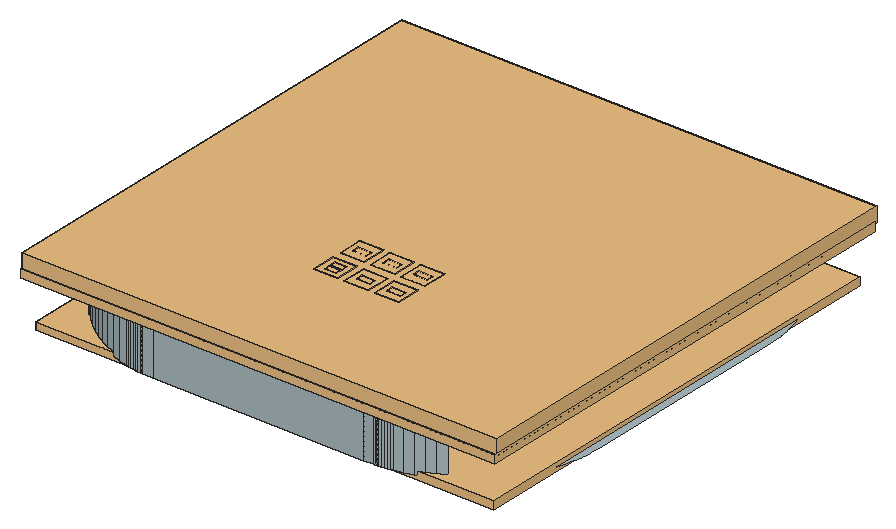
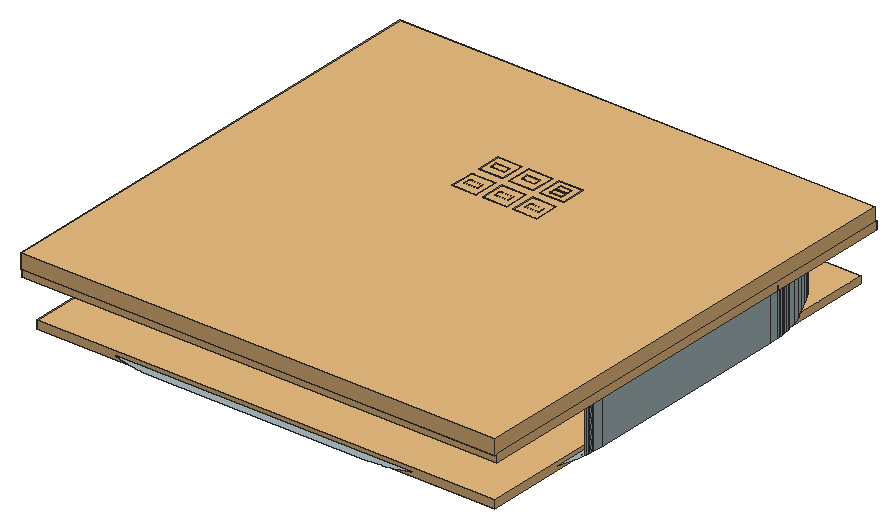
# SketchUp Ruby script. Lengths in inches.
U = 1.inch
M = Sketchup.active_model
def pt(a) = Geom::Point3d.new(a.map { |v| v * U })
def face(e, loops, mat)
  f = e.add_face(loops[0].map { |a| pt(a) })
  loops[1..].each { |l| e.add_face(l.map { |a| pt(a) }).erase! }
  f.material = f.back_material = mat if mat
  f
end
# faces: each face lists its corners as indices into pts; further lists are holes
def faces(e, pts, list, mat = nil) = list.each { |f| face(e, (f[0].is_a?(Array) ? f : [f]).map { |l| l.map { |i| pts[i] } }, mat) }
# xy, xz, yz: faces in a plane at the given z, y or x. An outline is a flat list of corners, or four numbers for a rectangle; further outlines are holes
def ring(l) = l.size == 4 ? [[l[0], l[1]], [l[2], l[1]], [l[2], l[3]], [l[0], l[3]]] : l.each_slice(2).to_a
def flat(e, list, mat, &to3) = list.each { |f| face(e, (f[0].is_a?(Array) ? f : [f]).map { |l| ring(l).map { |u, v| to3.(u, v) } }, mat) }
def xy(e, z, list, mat = nil) = flat(e, list, mat) { |x, y| [x, y, z] }
def xz(e, y, list, mat = nil) = flat(e, list, mat) { |x, z| [x, y, z] }
def yz(e, x, list, mat = nil) = flat(e, list, mat) { |y, z| [x, y, z] }
def lines(e, pts, list) = list.each { |a, b| e.add_line(pt(pts[a]), pt(pts[b])) }
# prism: a flat outline (further loops are holes) pulled along v
def prism(e, loops, v, mat = nil)
  f = face(e, loops, mat); d = Geom::Vector3d.new(v.map { |x| x * U })
  f.pushpull(f.normal.samedirection?(d) ? d.length : -d.length)
end
def box(e, o, s, mat = nil) = prism(e, [[o, [o[0] + s[0], o[1], o[2]], [o[0] + s[0], o[1] + s[1], o[2]], [o[0], o[1] + s[1], o[2]]]], [0, 0, s[2]], mat)
def at(x, y, z, deg = 0) = Geom::Transformation.translation(pt([x, y, z])) * Geom::Transformation.rotation(ORIGIN, Z_AXIS, deg.degrees)
def axes(o, x, y, z) = Geom::Transformation.new([*x, 0, *y, 0, *z, 0, *pt(o).to_a, 1])
def part(name) = M.definitions.add(name)
# library, detail: a bought-in or finely detailed component or shape, given as its bounding box
def library(name, o, s) = part(name).tap { |d| box(d.entities, o, s) }
def detail(e, o, s) = box(e.add_group.entities, o, s)
def put(e, d, t, mat = nil) = e.add_instance(d, t).tap { |i| i.material = mat if mat }
def group(e, t, mat = nil) = e.add_group.tap { |g| g.transformation = t; g.material = mat if mat }.entities
root = M.entities
M.materials.add("11").color = [255, 255, 255]
M.materials.add("26").color = [169, 186, 191]
c1 = library("Group103",[37538.96,7398.86,1636.89],[6.69,3.33,0.23])
c2 = library("Group97",[37538.89,7403.08,1636.87],[6.82,3.31,0.23])
c3 = library("Group98",[37538.36,7420.16,1636.8],[7.89,3.87,0.23])
c4 = library("om.cn_51",[-14089.91,-120000,166752.75],[16176.5,10000,4589.03])
c5 = library("om.cn_51698238",[-12277.97,-120000,175247.47],[24687.75,10000,11950.5])
c6 = library("Group104",[37556.32,7400.57,1636.88],[7.75,3.92,0.23])
c7 = library("Group99",[37556.29,7420.12,1636.8],[7.81,3.89,0.23])
c8 = library("Group113",[-159,-159,0],[318,318,8.4])
c9 = library("Group111",[-148.91,-148.91,209.88],[297.82,297.82,5])
c10 = library("Group59",[-149.91,-149.91,265.34],[299.82,299.82,4.68])
c11 = library("om.cn_51268574",[-7425.4375,-120000,166763.1875],[21515.3125,10000,4564.15])
c12 = library("Group105",[37574.14,7400.59,1636.88],[7.9,3.89,0.23])
c13 = library("Group101",[37574.11,7420.12,1636.8],[7.96,3.91,0.23])
xy(root,90.6622,[[[290.4563,4.7461,290.2394,4.7537,290.2089,4.756,290.1785,4.7586,290.148,4.7615,290.1176,4.7648,290.0873,4.7683,290.0569,4.7721,290.0266,4.7763,289.9968,4.7806,289.9669,4.7853,289.9371,4.7903,289.9074,4.7956,289.8777,4.8012,289.848,4.8071,289.8185,4.8133,289.6154,4.8641,289.418,4.9284,289.2268,5.0055,289.0422,5.095,288.8648,5.1964,288.6951,5.309,288.5336,5.4324,288.3809,5.5662,288.2374,5.7097,288.1036,5.8624,287.9802,6.0239,287.8676,6.1936,287.7662,6.371,287.6768,6.5556,287.5996,6.7468,287.5353,6.9442,287.4845,7.1473,287.4783,7.1768,287.4724,7.2065,287.4668,7.2362,287.4615,7.2659,287.4565,7.2957,287.4519,7.3255,287.4475,7.3554,287.4433,7.3857,287.4395,7.4161,287.436,7.4464,287.4327,7.4768,287.4298,7.5073,287.4272,7.5377,287.4249,7.5682,287.4173,7.7851,287.4173,12.6889,287.4249,12.9057,287.4272,12.9362,287.4298,12.9667,287.4327,12.9971,287.436,13.0275,287.4395,13.0579,287.4433,13.0882,287.4475,13.1185,287.4519,13.1484,287.4565,13.1782,287.4615,13.208,287.4668,13.2378,287.4724,13.2675,287.4783,13.2971,287.4845,13.3267,287.5353,13.5297,287.5996,13.7271,287.6768,13.9184,287.7662,14.103,287.8676,14.2804,287.9802,14.4501,288.1036,14.6115,288.2374,14.7643,288.3809,14.9078,288.5336,15.0415,288.6951,15.1649,288.8648,15.2776,289.0422,15.3789,289.2268,15.4684,289.418,15.5455,289.6154,15.6098,289.8185,15.6607,289.848,15.6669,289.8777,15.6727,289.9074,15.6783,289.9371,15.6836,289.9669,15.6886,289.9968,15.6933,290.0266,15.6977,290.0569,15.7018,290.0873,15.7056,290.1176,15.7092,290.148,15.7124,290.1785,15.7153,290.2089,15.7179,290.2394,15.7202,290.4563,15.7279,295.3601,15.7279,295.5769,15.7202,295.6074,15.7179,295.6379,15.7153,295.6683,15.7124,295.6987,15.7092,295.7291,15.7056,295.7594,15.7018,295.7897,15.6977,295.8196,15.6933,295.8494,15.6886,295.8792,15.6836,295.909,15.6783,295.9387,15.6727,295.9683,15.6669,295.9979,15.6607,296.2009,15.6098,296.3983,15.5455,296.5896,15.4684,296.7742,15.3789,296.9516,15.2776,297.1213,15.1649,297.2827,15.0415,297.4355,14.9078,297.579,14.7643,297.7127,14.6115,297.8361,14.4501,297.9488,14.2804,298.0501,14.103,298.1396,13.9184,298.2167,13.7271,298.281,13.5297,298.3319,13.3267,298.3381,13.2971,298.3439,13.2675,298.3495,13.2378,298.3548,13.208,298.3598,13.1782,298.3645,13.1484,298.3689,13.1185,298.373,13.0882,298.3768,13.0579,298.3804,13.0275,298.3836,12.9971,298.3865,12.9667,298.3891,12.9362,298.3915,12.9057,298.3991,12.6889,298.3991,7.7851,298.3914,7.5682,298.3891,7.5377,298.3865,7.5073,298.3836,7.4768,298.3804,7.4464,298.3768,7.4161,298.373,7.3857,298.3689,7.3554,298.3645,7.3255,298.3598,7.2957,298.3548,7.2659,298.3495,7.2362,298.3439,7.2065,298.3381,7.1768,298.3319,7.1473,298.281,6.9442,298.2167,6.7468,298.1396,6.5556,298.0501,6.371,297.9488,6.1936,297.8361,6.0239,297.7127,5.8624,297.579,5.7097,297.4355,5.5662,297.2827,5.4324,297.1213,5.309,296.9516,5.1964,296.7742,5.095,296.5896,5.0055,296.3983,4.9284,296.2009,4.8641,295.9979,4.8133,295.9683,4.8071,295.9387,4.8012,295.909,4.7956,295.8792,4.7903,295.8494,4.7853,295.8196,4.7806,295.7897,4.7763,295.7594,4.7721,295.7291,4.7683,295.6987,4.7648,295.6683,4.7615,295.6379,4.7586,295.6074,4.756,295.5769,4.7537,295.3601,4.7461],[287.484,13.1133,287.5204,13.3184,287.5144,13.2897,287.484,13.1133,287.4979,13.2018,287.4929,13.1723,287.4883,13.1428]]],"26")
xy(root,91.8361,[[[290.4563,4.7461,295.3601,4.7461,295.5769,4.7537,295.6074,4.756,295.6379,4.7586,295.6683,4.7615,295.6987,4.7648,295.7291,4.7683,295.7594,4.7721,295.7897,4.7763,295.8196,4.7806,295.8494,4.7853,295.8792,4.7903,295.909,4.7956,295.9387,4.8012,295.9683,4.8071,295.9979,4.8133,296.2009,4.8641,296.3983,4.9284,296.5896,5.0055,296.7742,5.095,296.9516,5.1964,297.1213,5.309,297.2827,5.4324,297.4355,5.5662,297.579,5.7097,297.7127,5.8624,297.8361,6.0239,297.9488,6.1936,298.0501,6.371,298.1396,6.5556,298.2167,6.7468,298.281,6.9442,298.3319,7.1473,298.3381,7.1768,298.3439,7.2065,298.3495,7.2362,298.3548,7.2659,298.3598,7.2957,298.3645,7.3255,298.3689,7.3554,298.373,7.3857,298.3768,7.4161,298.3804,7.4464,298.3836,7.4768,298.3865,7.5073,298.3891,7.5377,298.3914,7.5682,298.3991,7.7851,298.3991,12.6889,298.3915,12.9057,298.3891,12.9362,298.3865,12.9667,298.3836,12.9971,298.3804,13.0275,298.3768,13.0579,298.373,13.0882,298.3689,13.1185,298.3645,13.1484,298.3598,13.1782,298.3548,13.208,298.3495,13.2378,298.3439,13.2675,298.3381,13.2971,298.3319,13.3267,298.281,13.5297,298.2167,13.7271,298.1396,13.9184,298.0501,14.103,297.9488,14.2804,297.8361,14.4501,297.7127,14.6115,297.579,14.7643,297.4355,14.9078,297.2827,15.0415,297.1213,15.1649,296.9516,15.2776,296.7742,15.3789,296.5896,15.4684,296.3983,15.5455,296.2009,15.6098,295.9979,15.6607,295.9683,15.6669,295.9387,15.6727,295.909,15.6783,295.8792,15.6836,295.8494,15.6886,295.8196,15.6933,295.7897,15.6977,295.7594,15.7018,295.7291,15.7056,295.6987,15.7092,295.6683,15.7124,295.6379,15.7153,295.6074,15.7179,295.5769,15.7202,295.3601,15.7279,290.4563,15.7279,290.2394,15.7202,290.2089,15.7179,290.1785,15.7153,290.148,15.7124,290.1176,15.7092,290.0873,15.7056,290.0569,15.7018,290.0266,15.6977,289.9968,15.6933,289.9669,15.6886,289.9371,15.6836,289.9074,15.6783,289.8777,15.6727,289.848,15.6669,289.8185,15.6607,289.6154,15.6098,289.418,15.5455,289.2268,15.4684,289.0422,15.3789,288.8648,15.2776,288.6951,15.1649,288.5336,15.0415,288.3809,14.9078,288.2374,14.7643,288.1036,14.6115,287.9802,14.4501,287.8676,14.2804,287.7662,14.103,287.6768,13.9184,287.5996,13.7271,287.5353,13.5297,287.4845,13.3267,287.4783,13.2971,287.4724,13.2675,287.4668,13.2378,287.4615,13.208,287.4565,13.1782,287.4519,13.1484,287.4475,13.1185,287.4433,13.0882,287.4395,13.0579,287.436,13.0275,287.4327,12.9971,287.4298,12.9667,287.4272,12.9362,287.4249,12.9057,287.4173,12.6889,287.4173,7.7851,287.4249,7.5682,287.4272,7.5377,287.4298,7.5073,287.4327,7.4768,287.436,7.4464,287.4395,7.4161,287.4433,7.3857,287.4475,7.3554,287.4519,7.3255,287.4565,7.2957,287.4615,7.2659,287.4668,7.2362,287.4724,7.2065,287.4783,7.1768,287.4845,7.1473,287.5353,6.9442,287.5996,6.7468,287.6768,6.5556,287.7662,6.371,287.8676,6.1936,287.9802,6.0239,288.1036,5.8624,288.2374,5.7097,288.3809,5.5662,288.5336,5.4324,288.6951,5.309,288.8648,5.1964,289.0422,5.095,289.2268,5.0055,289.418,4.9284,289.6154,4.8641,289.8185,4.8133,289.848,4.8071,289.8777,4.8012,289.9074,4.7956,289.9371,4.7903,289.9669,4.7853,289.9968,4.7806,290.0266,4.7763,290.0569,4.7721,290.0873,4.7683,290.1176,4.7648,290.148,4.7615,290.1785,4.7586,290.2089,4.756,290.2394,4.7537],[287.5647,7.1657,287.559,7.1933,287.5533,7.2221,287.5478,7.251,287.5427,7.2799,287.5333,7.3379,287.529,7.367,287.525,7.3965,287.5212,7.426,287.5178,7.4555,287.5147,7.4851,287.5118,7.5147,287.5093,7.5443,287.5071,7.5727,287.5118,7.5147,287.525,7.3965,287.5427,7.2799,287.5533,7.2221],[298.3092,12.9012,298.3045,12.9592,298.2914,13.0775,298.2737,13.194,298.2631,13.2518,298.2516,13.3082,298.2574,13.2807,298.2631,13.2518,298.2685,13.223,298.2737,13.194,298.2831,13.136,298.2873,13.107,298.2914,13.0775,298.2951,13.048,298.2985,13.0184,298.3017,12.9888,298.3045,12.9592,298.3071,12.9296],[289.8369,15.5804,289.8645,15.5862,289.8933,15.5919,289.9222,15.5973,289.9511,15.6025,290.0091,15.6119,290.0382,15.6161,290.0677,15.6202,290.0972,15.6239,290.1267,15.6273,290.1563,15.6305,290.1859,15.6333,290.2155,15.6359,290.244,15.638,290.1859,15.6333,290.0677,15.6202,289.9511,15.6025,289.8933,15.5919],[295.5724,4.8359,295.6304,4.8406,295.7487,4.8538,295.8652,4.8715,295.923,4.8821,295.9794,4.8935,295.9519,4.8878,295.923,4.8821,295.8942,4.8766,295.8652,4.8715,295.8072,4.8621,295.7782,4.8578,295.7487,4.8538,295.7192,4.85,295.6896,4.8466,295.66,4.8435,295.6304,4.8406,295.6008,4.8381],[298.2685,7.251,298.2785,7.3089,298.2873,7.367,298.2951,7.426,298.3017,7.4851,298.3071,7.5443,298.3045,7.5147,298.3017,7.4851,298.2985,7.4555,298.2951,7.426,298.2914,7.3965,298.2873,7.367,298.2831,7.3379,298.2785,7.3089,298.2737,7.2799],[287.5093,12.9296,287.5118,12.9592,287.5147,12.9888,287.5178,13.0184,287.5212,13.048,287.525,13.0775,287.529,13.107,287.5333,13.136,287.5378,13.165,287.5427,13.194,287.5478,13.223,287.5378,13.165,287.529,13.107,287.5212,13.048,287.5147,12.9888],[295.8942,15.5973,295.8362,15.6073,295.7782,15.6161,295.7192,15.6239,295.66,15.6305,295.6008,15.6359,295.6304,15.6333,295.66,15.6305,295.6896,15.6273,295.7192,15.6239,295.7487,15.6202,295.7782,15.6161,295.8072,15.6119,295.8362,15.6073,295.8652,15.6025],[290.2155,4.8381,290.1859,4.8406,290.1563,4.8435,290.1267,4.8466,290.0972,4.85,290.0677,4.8538,290.0382,4.8578,290.0091,4.8621,289.9801,4.8666,289.9511,4.8715,289.9222,4.8766,289.9801,4.8666,290.0382,4.8578,290.0972,4.85,290.1563,4.8435]],[295.5724,4.8359,295.6008,4.8381,295.6304,4.8406],[290.2155,4.8381,290.1563,4.8435,290.1859,4.8406],[295.6304,4.8406,295.66,4.8435,295.6896,4.8466,295.7487,4.8538],[290.1563,4.8435,290.0972,4.85,290.1267,4.8466],
  [295.6896,4.8466,295.7192,4.85,295.7487,4.8538],[290.0972,4.85,290.0382,4.8578,290.0677,4.8538],[295.7487,4.8538,295.7782,4.8578,295.8072,4.8621],[295.7487,4.8538,295.8072,4.8621,295.8652,4.8715],[290.0382,4.8578,289.9801,4.8666,290.0091,4.8621],
  [289.9801,4.8666,289.9222,4.8766,289.9511,4.8715],[295.8652,4.8715,295.8942,4.8766,295.923,4.8821],[295.923,4.8821,295.9519,4.8878,295.9794,4.8935],[287.5647,7.1657,287.5533,7.2221,287.559,7.1933],[287.5533,7.2221,287.5427,7.2799,287.5478,7.251],
  [287.5427,7.2799,287.525,7.3965,287.5333,7.3379],[287.5333,7.3379,287.525,7.3965,287.529,7.367],[287.525,7.3965,287.5118,7.5147,287.5147,7.4851,287.5178,7.4555],[287.525,7.3965,287.5178,7.4555,287.5212,7.426],[287.5118,7.5147,287.5071,7.5727,287.5093,7.5443],
  [287.5093,12.9296,287.5147,12.9888,287.5118,12.9592],[287.5147,12.9888,287.5212,13.048,287.5178,13.0184],[287.5212,13.048,287.529,13.107,287.525,13.0775]],"26")
xz(root,4.7461,[[290.4563,90.6622,295.3601,91.8361]],"26")
yz(root,287.4173,[[7.7851,90.6622,12.6889,91.8361]],"26")
p = [[290.4563,4.7461,90.6622],[290.4563,4.7461,91.8361],[290.2394,4.7537,91.8361],[290.2394,4.7537,90.6622],[295.5769,4.7537,90.6622],[295.5769,4.7537,91.8361],
  [295.3601,4.7461,91.8361],[295.3601,4.7461,90.6622],[289.8185,4.8133,90.6622],[289.8185,4.8133,91.8361],[289.6154,4.8641,91.8361],[289.6154,4.8641,90.6622],
  [289.848,4.8071,90.6622],[289.848,4.8071,91.8361],[289.8777,4.8012,90.6622],[289.8777,4.8012,91.8361],[289.9074,4.7956,90.6622],[289.9074,4.7956,91.8361],
  [289.9371,4.7903,90.6622],[289.9371,4.7903,91.8361],[289.9669,4.7853,90.6622],[289.9669,4.7853,91.8361],[289.9968,4.7806,90.6622],[289.9968,4.7806,91.8361],
  [290.0266,4.7763,90.6622],[290.0266,4.7763,91.8361],[290.0569,4.7721,90.6622],[290.0569,4.7721,91.8361],[290.0873,4.7683,90.6622],[290.0873,4.7683,91.8361],
  [290.1176,4.7648,90.6622],[290.1176,4.7648,91.8361],[290.148,4.7615,90.6622],[290.148,4.7615,91.8361],[290.1785,4.7586,90.6622],[290.1785,4.7586,91.8361],
  [290.2089,4.756,90.6622],[290.2089,4.756,91.8361],[295.6074,4.756,90.6622],[295.6074,4.756,91.8361],[295.6379,4.7586,90.6622],[295.6379,4.7586,91.8361],
  [295.6683,4.7615,90.6622],[295.6683,4.7615,91.8361],[295.6987,4.7648,90.6622],[295.6987,4.7648,91.8361],[295.7291,4.7683,90.6622],[295.7291,4.7683,91.8361],
  [295.7594,4.7721,90.6622],[295.7594,4.7721,91.8361],[295.7897,4.7763,90.6622],[295.7897,4.7763,91.8361],[295.8196,4.7806,90.6622],[295.8196,4.7806,91.8361],
  [295.8494,4.7853,90.6622],[295.8494,4.7853,91.8361],[295.8792,4.7903,90.6622],[295.8792,4.7903,91.8361],[295.909,4.7956,90.6622],[295.909,4.7956,91.8361],
  [295.9387,4.8012,90.6622],[295.9387,4.8012,91.8361],[295.9683,4.8071,90.6622],[295.9683,4.8071,91.8361],[295.9979,4.8133,90.6622],[295.9979,4.8133,91.8361],
  [296.2009,4.8641,90.6622],[296.2009,4.8641,91.8361],[289.418,4.9284,90.6622],[289.418,4.9284,91.8361],[289.2268,5.0055,91.8361],[289.2268,5.0055,90.6622],
  [296.3983,4.9284,90.6622],[296.3983,4.9284,91.8361],[296.5896,5.0055,90.6622],[296.5896,5.0055,91.8361],[289.0422,5.095,91.8361],[289.0422,5.095,90.6622],
  [296.7742,5.095,90.6622],[296.7742,5.095,91.8361],[288.8648,5.1964,91.8361],[288.8648,5.1964,90.6622],[296.9516,5.1964,90.6622],[296.9516,5.1964,91.8361],
  [288.6951,5.309,91.8361],[288.6951,5.309,90.6622],[288.5336,5.4324,91.8361],[288.5336,5.4324,90.6622],[288.3809,5.5662,91.8361],[288.3809,5.5662,90.6622],
  [288.2374,5.7097,91.8361],[288.2374,5.7097,90.6622],[288.1036,5.8624,91.8361],[288.1036,5.8624,90.6622],[287.9802,6.0239,91.8361],[287.9802,6.0239,90.6622],
  [287.8676,6.1936,91.8361],[287.8676,6.1936,90.6622],[287.7662,6.371,91.8361],[287.7662,6.371,90.6622],[287.6768,6.5556,91.8361],[287.6768,6.5556,90.6622],
  [287.5996,6.7468,91.8361],[287.5996,6.7468,90.6622],[287.5353,6.9442,91.8361],[287.5353,6.9442,90.6622],[287.4845,7.1473,91.8361],[287.4845,7.1473,90.6622],
  [287.4783,7.1768,91.8361],[287.4783,7.1768,90.6622],[287.4668,7.2362,90.6622],[287.4668,7.2362,91.8361],[287.4615,7.2659,91.8361],[287.4615,7.2659,90.6622],
  [287.4724,7.2065,90.6622],[287.4724,7.2065,91.8361],[287.4519,7.3255,90.6622],[287.4519,7.3255,91.8361],[287.4475,7.3554,91.8361],[287.4475,7.3554,90.6622],
  [287.4565,7.2957,90.6622],[287.4565,7.2957,91.8361],[287.436,7.4464,90.6622],[287.436,7.4464,91.8361],[287.4327,7.4768,91.8361],[287.4327,7.4768,90.6622],
  [287.4395,7.4161,90.6622],[287.4395,7.4161,91.8361],[287.4433,7.3857,90.6622],[287.4433,7.3857,91.8361],[287.4272,7.5377,90.6622],[287.4272,7.5377,91.8361],
  [287.4249,7.5682,91.8361],[287.4249,7.5682,90.6622],[287.4298,7.5073,90.6622],[287.4298,7.5073,91.8361],[287.4173,7.7851,91.8361],[287.4173,7.7851,90.6622],
  [287.4173,12.6889,90.6622],[287.4173,12.6889,91.8361],[287.4249,12.9057,91.8361],[287.4249,12.9057,90.6622],[287.4272,12.9362,91.8361],[287.4272,12.9362,90.6622],
  [287.4298,12.9667,91.8361],[287.4298,12.9667,90.6622],[287.4327,12.9971,91.8361],[287.4327,12.9971,90.6622],[287.436,13.0275,91.8361],[287.436,13.0275,90.6622],
  [287.4395,13.0579,91.8361],[287.4395,13.0579,90.6622],[287.4433,13.0882,91.8361],[287.4433,13.0882,90.6622],[287.4475,13.1185,91.8361],[287.4475,13.1185,90.6622]]
faces(root,p,[[0,1,2,3],[4,5,6,7],[8,9,10,11],[12,13,9,8],[14,15,13,12],[16,17,15,14],[18,19,17,16],[20,21,19,18],
  [22,23,21,20],[24,25,23,22],[26,27,25,24],[28,29,27,26],[30,31,29,28],[32,33,31,30],[34,35,33,32],[36,37,35,34],
  [3,2,37,36],[38,39,5,4],[40,41,39,38],[42,43,41,40],[44,45,43,42],[46,47,45,44],[48,49,47,46],[50,51,49,48],
  [52,53,51,50],[54,55,53,52],[56,57,55,54],[58,59,57,56],[60,61,59,58],[62,63,61,60],[64,65,63,62],[66,67,65,64],
  [68,69,70,71],[11,10,69,68],[72,73,67,66],[74,75,73,72],[71,70,76,77],[78,79,75,74],[77,76,80,81],[82,83,79,78],
  [81,80,84,85],[85,84,86,87],[87,86,88,89],[89,88,90,91],[91,90,92,93],[93,92,94,95],[95,94,96,97],[97,96,98,99],
  [99,98,100,101],[101,100,102,103],[103,102,104,105],[105,104,106,107],[107,106,108,109],[110,111,112,113],[114,115,111,110],[109,108,115,114],
  [116,117,118,119],[120,121,117,116],[113,112,121,120],[122,123,124,125],[126,127,123,122],[128,129,127,126],[119,118,129,128],[130,131,132,133],
  [134,135,131,130],[125,124,135,134],[133,132,136,137],[138,139,140,141],[141,140,142,143],[143,142,144,145],[145,144,146,147],[147,146,148,149],
  [149,148,150,151],[151,150,152,153],[153,152,154,155]],"26")
g1 = group(root,at(-1185.85,-283.55,27.72))
detail(g1,[1477.76,291.16,64.44],[0.55,0.56,0.01])
g2 = group(root,at(-1185.85,-283.55,27.72))
detail(g2,[1477.76,291.93,64.44],[0.55,0.56,0.01])
put(root,c1,axes([-1185.85,-283.55,27.72],[0.03937,0,0],[0,0.03937,0],[0,0,0.03937]))
put(root,c2,axes([-1185.85,-283.55,27.72],[0.03937,0,0],[0,0.03937,0],[0,0,0.03937]))
put(root,c3,axes([-1185.85,-283.55,27.72],[0.03937,0,0],[0,0.03937,0],[0,0,0.03937]))
put(root,c4,axes([292.89,-7.22,93.125],[0.00008,0,0],[0,0,0.00001],[0,0.00008,0]),"11")
put(root,c5,axes([292.86,-0.37,93.1],[0.00005,0,0],[0,0,0.00001],[0,0.00005,0]),"11")
g3 = group(root,at(-1185.85,-283.55,27.72))
detail(g3,[1478.46,291.16,64.44],[0.56,0.56,0.01])
g4 = group(root,at(-1185.85,-283.55,27.72))
detail(g4,[1478.46,291.93,64.44],[0.56,0.56,0.01])
put(root,c6,axes([-1185.85,-283.55,27.72],[0.03937,0,0],[0,0.03937,0],[0,0,0.03937]))
put(root,c7,axes([-1185.85,-283.55,27.72],[0.03937,0,0],[0,0.03937,0],[0,0,0.03937]))
put(root,c8,axes([292.91,10.27,91.83],[0.03459,0,0],[0,0.03459,0],[0,0,0.04047]))
put(root,c9,axes([292.91,10.24,82.82],[0.03558,0,0],[0,0.03558,0],[0,0,0.03687]))
put(root,c10,axes([292.91,10.24,80.6875],[0.03669,0,0],[0,0.03669,0],[0,0,0.04136]))
put(root,c11,axes([292.89,-7.22,93.125],[0.00008,0,0],[0,0,0.00001],[0,0.00008,0]),"11")
g5 = group(root,at(-1185.85,-283.55,27.72))
detail(g5,[1479.17,291.16,64.44],[0.55,0.56,0.01])
g6 = group(root,at(-1185.85,-283.55,27.72))
detail(g6,[1479.17,291.93,64.44],[0.55,0.56,0.01])
put(root,c12,axes([-1185.85,-283.55,27.72],[0.03937,0,0],[0,0.03937,0],[0,0,0.03937]))
put(root,c13,axes([-1185.85,-283.55,27.72],[0.03937,0,0],[0,0.03937,0],[0,0,0.03937]))
